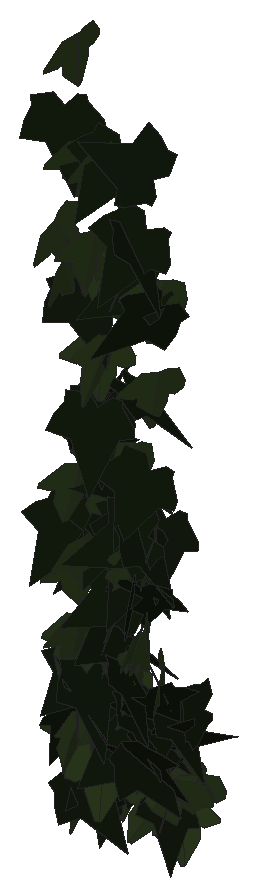
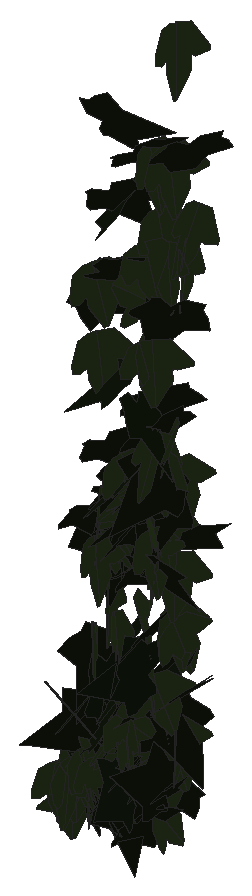
# SketchUp Ruby script. Lengths in inches.
U = 1.inch
M = Sketchup.active_model
def pt(a) = Geom::Point3d.new(a.map { |v| v * U })
def face(e, loops, mat)
  f = e.add_face(loops[0].map { |a| pt(a) })
  loops[1..].each { |l| e.add_face(l.map { |a| pt(a) }).erase! }
  f.material = f.back_material = mat if mat
  f
end
# faces: each face lists its corners as indices into pts; further lists are holes
def faces(e, pts, list, mat = nil) = list.each { |f| face(e, (f[0].is_a?(Array) ? f : [f]).map { |l| l.map { |i| pts[i] } }, mat) }
# xy, xz, yz: faces in a plane at the given z, y or x. An outline is a flat list of corners, or four numbers for a rectangle; further outlines are holes
def ring(l) = l.size == 4 ? [[l[0], l[1]], [l[2], l[1]], [l[2], l[3]], [l[0], l[3]]] : l.each_slice(2).to_a
def flat(e, list, mat, &to3) = list.each { |f| face(e, (f[0].is_a?(Array) ? f : [f]).map { |l| ring(l).map { |u, v| to3.(u, v) } }, mat) }
def xy(e, z, list, mat = nil) = flat(e, list, mat) { |x, y| [x, y, z] }
def xz(e, y, list, mat = nil) = flat(e, list, mat) { |x, z| [x, y, z] }
def yz(e, x, list, mat = nil) = flat(e, list, mat) { |y, z| [x, y, z] }
def lines(e, pts, list) = list.each { |a, b| e.add_line(pt(pts[a]), pt(pts[b])) }
# prism: a flat outline (further loops are holes) pulled along v
def prism(e, loops, v, mat = nil)
  f = face(e, loops, mat); d = Geom::Vector3d.new(v.map { |x| x * U })
  f.pushpull(f.normal.samedirection?(d) ? d.length : -d.length)
end
def box(e, o, s, mat = nil) = prism(e, [[o, [o[0] + s[0], o[1], o[2]], [o[0] + s[0], o[1] + s[1], o[2]], [o[0], o[1] + s[1], o[2]]]], [0, 0, s[2]], mat)
def at(x, y, z, deg = 0) = Geom::Transformation.translation(pt([x, y, z])) * Geom::Transformation.rotation(ORIGIN, Z_AXIS, deg.degrees)
def axes(o, x, y, z) = Geom::Transformation.new([*x, 0, *y, 0, *z, 0, *pt(o).to_a, 1])
def part(name) = M.definitions.add(name)
# library, detail: a bought-in or finely detailed component or shape, given as its bounding box
def library(name, o, s) = part(name).tap { |d| box(d.entities, o, s) }
def detail(e, o, s) = box(e.add_group.entities, o, s)
def put(e, d, t, mat = nil) = e.add_instance(d, t).tap { |i| i.material = mat if mat }
def group(e, t, mat = nil) = e.add_group.tap { |g| g.transformation = t; g.material = mat if mat }.entities
root = M.entities
M.materials.add("efeu1").color = [18, 25, 13]
M.materials.add("efeu2").color = [43, 57, 29]
c1 = part("ivyleaf_9")
p = [[1.54,2.16,1.25],[1.36,2.04,1.19],[-0.21,0.99,0.68],[-0.71,1.11,0.82],[-0.85,0.86,0.67],[-0.8,0.17,0.21],
  [-0.9,-0.01,0.1],[-0.67,-0.16,-0.02],[-0.08,-0.08,-0.05],[-0.03,-0.6,-0.4],[0.65,-0.88,-0.66],[0.83,-0.6,-0.49],
  [1.29,-0.42,-0.43],[1.8125,-0.07,-0.26],[1.21,0.44,0.15]]
faces(c1.entities,p,[[0,1,2,3,4,5,6,7,8,9,10,11,12,13,14]],"efeu1")
c2 = part("ivyleaf_10")
p = [[0,0.5,-0.03],[-0.0625,2.02,-0.43],[-0.19,2.01,-0.46],[-0.54,1.05,-0.29],[-0.52,0.625,-0.18],[-0.83,0.76,-0.28],
  [-1.16,0.64,-0.33],[-1.15,0.33,-0.24],[-0.77,-0.39,0.02],[-0.3,-0.51,0.16],[0.04,-0.48,0.23],[-0.02,2.01,-0.4375],
  [-0.06,2.01,-0.43],[0.04,-0.49,0.23],[0.67,-0.49,0.14],[1.38,0.36,-0.2],[1.375,0.51,-0.24],[0.81,0.65,-0.19],
  [0.62,0.59,-0.15],[0.6,1.09,-0.28],[0.5,1.23,-0.31]]
faces(c2.entities,p,[[0,1,2,3,4,5,6,7,8,9,10],[11,12,0,13,14,15,16,17,18,19,20]],"efeu2")
put(root,c1,axes([534.67,132.68,230.73],[-0.17047,-0.87063,-0.31313],[0.13235,0.29218,-0.88443],[0.91571,-0.2043,0.06954]))
put(root,c1,axes([535,132.6,216.09],[-0.49505,-0.70564,0.21497],[-0.01913,-0.24653,-0.85327],[0.73741,-0.48012,0.12218]))
put(root,c1,axes([534.84,133.875,207.48],[0.16353,0.01722,0.84757],[0.46903,0.71721,-0.10507],[-0.70617,0.48035,0.12649]))
put(root,c1,axes([535,133.2,210.3125],[-0.40753,-0.58007,0.50539],[-0.0202,-0.56365,-0.66322],[0.76908,-0.32218,0.25038]))
put(root,c2,axes([535.21,133.21,219.01],[-0.87167,0.19635,0.09667],[-0.12722,-0.13155,-0.8799],[-0.17809,-0.86709,0.15539]))
put(root,c2,axes([534.99,133.64,206.32],[0.17022,-0.68568,0.54442],[0.19711,-0.51036,-0.70442],[0.85305,0.25475,0.05413]))
put(root,c2,axes([535.3,133.59,210.88],[-0.51327,-0.62942,0.32203],[-0.08648,-0.33906,-0.80055],[0.70171,-0.50218,0.13689]))
put(root,c2,axes([535.08,133.01,220.08],[-0.46392,0.76914,-0.00582],[0.00287,-0.00506,-0.89822],[-0.76915,-0.46393,0.00015]))
put(root,c1,axes([535.41,132.59,209.51],[-0.00032,0.72675,-0.57082],[-0.0098,-0.5708,-0.7267],[-0.92407,0.00581,0.00791]))
put(root,c1,axes([535.11,134.04,206.78],[-0.27107,-0.63117,0.50294],[-0.07725,-0.50782,-0.67893],[0.80334,-0.26181,0.10441]))
put(root,c2,axes([535.51,132.76,208.73],[-0.64757,-0.66757,0.33135],[-0.19199,-0.27473,-0.92868],[0.72012,-0.67355,0.05038]))
put(root,c2,axes([535.35,133.72,216.23],[-0.13916,-0.88516,0.00004],[-0.00327,0.00047,-0.89602],[0.88515,-0.13916,-0.0033]))
put(root,c2,axes([535.4,132.28,208.78],[0.28299,-0.69072,-0.55775],[-0.1092,0.55387,-0.74132],[0.88105,0.2905,0.08727]))
put(root,c2,axes([535.33,132.43,212.42],[-0.20741,-0.77307,0.34276],[0.12229,-0.37663,-0.77545],[0.83676,-0.13658,0.19829]))
put(root,c1,axes([535.66,133.65,215.38],[-0.88423,-0.15992,-0.0197],[0.02107,-0.00578,-0.89853],[0.15975,-0.88443,0.00944]))
put(root,c2,axes([535.44,132.39,214.8125],[-0.42454,-0.77265,-0.09329],[0.03674,0.08625,-0.88156],[0.7774,-0.42603,-0.00928]))
put(root,c2,axes([535.34,131.5,227.28],[-0.08329,-0.81917,-0.55725],[0.1681,0.53942,-0.81809],[0.97638,-0.16275,0.09331]))
put(root,c1,axes([535.25,134.5,206.3],[-0.23027,-0.82502,0.03105],[-0.00851,-0.02986,-0.85655],[0.82556,-0.23043,-0.00017]))
put(root,c2,axes([535.54,132.21,218.11],[-0.34714,-0.81372,0.16705],[-0.036,-0.16614,-0.88411],[0.82991,-0.34758,0.03152]))
put(root,c1,axes([535.08,133.37,218.73],[0.80409,0.42348,0.0933],[0.09341,0.02278,-0.90849],[-0.42345,0.80917,-0.02325]))
put(root,c2,axes([535.59,132.48,229.77],[-0.32626,-0.89624,0.01194],[-0.00363,-0.01139,-0.95378],[0.89631,-0.32628,0.00049]))
put(root,c2,axes([535.53,133.26,215.76],[0.43509,-0.63287,-0.47452],[-0.04953,0.51871,-0.73722],[0.78946,0.38133,0.21527]))
put(root,c2,axes([535.55,131.54,225.99],[0.22422,-0.76891,-0.52224],[-0.01101,0.53498,-0.79241],[0.92943,0.19184,0.1166]))
put(root,c2,axes([535.58,132.16,212.76],[-0.13049,-0.88511,-0.01911],[0.001,0.01917,-0.89468],[0.88532,-0.13048,-0.0018]))
put(root,c2,axes([535.52,133.32,219.63],[-0.1619,-0.78602,-0.44335],[0.12954,0.42553,-0.80171],[0.89309,-0.20421,0.03592]))
put(root,c2,axes([535.53,133.54,217.13],[0.43022,-0.77724,0.17532],[0.07912,-0.15658,-0.88834],[0.79283,0.43738,-0.00648]))
put(root,c2,axes([535.91,132.37,226.08],[-0.85268,0.1476,0.327],[-0.33414,-0.01969,-0.8624],[-0.13064,-0.91302,0.07147]))
put(root,c1,axes([535.62,132.79,217.48],[0.66238,0.53861,-0.27147],[-0.244,-0.12946,-0.8522],[-0.5516,0.70405,0.05098]))
put(root,c2,axes([535.72,133.43,211.61],[0.51148,-0.64356,-0.29086],[-0.09639,0.29215,-0.81593],[0.69963,0.51074,0.10022]))
put(root,c1,axes([535.34,132.79,224.54],[-0.28565,-0.64315,-0.59252],[0.27511,0.52558,-0.70313],[0.83008,-0.39551,0.02914]))
put(root,c1,axes([535.8,134.68,207.38],[0.13468,0.46315,0.75382],[0.05072,0.7572,-0.4743],[-0.88328,0.1141,0.08771]))
put(root,c1,axes([536.08,133.48,220.95],[-0.52812,0.71989,-0.16553],[0.09619,-0.13473,-0.89283],[-0.73238,-0.5368,0.0021]))
put(root,c2,axes([535.81,131.86,233.93],[-0.1333,-0.94983,-0.2069],[0.02636,0.20523,-0.95914],[0.97175,-0.13586,-0.00236]))
put(root,c2,axes([535.95,134.45,209.92],[0.26425,0.58423,-0.62362],[-0.37411,-0.50779,-0.63424],[-0.76829,0.4482,0.09434]))
put(root,c2,axes([535.9375,134.1875,209.4],[0.56503,-0.5662,-0.32944],[-0.08799,0.36552,-0.77912],[0.64913,0.54239,0.18115]))
put(root,c1,axes([535.37,132.28,210.8],[0.50198,-0.68368,0.19339],[0.1189,-0.15261,-0.84816],[0.70049,0.51584,0.00538]))
put(root,c1,axes([535.66,133.22,220.25],[-0.08997,-0.9049,-0.15923],[-0.01163,0.1611,-0.90896],[0.91873,-0.08657,-0.0271]))
put(root,c1,axes([535.28,134.2,211.64],[0.81082,-0.25843,0.35026],[0.33924,-0.08882,-0.85084],[0.27273,0.87877,0.01701]))
put(root,c2,axes([535.58,132.89,209.71],[0.43676,-0.48327,0.57608],[0.50444,-0.30574,-0.63893],[0.55764,0.65509,0.12678]))
put(root,c2,axes([536.08,132.81,222.59],[-0.6913,-0.62824,0.08275],[0.06346,-0.19049,-0.91603],[0.63048,-0.66967,0.18293]))
put(root,c1,axes([536.3125,133.9375,206.54],[-0.0256,0.82399,-0.17062],[-0.01516,-0.17112,-0.82414],[-0.84133,-0.02199,0.02004]))
put(root,c1,axes([535.53,132.46,206.97],[-0.15224,-0.36617,-0.83759],[0.6488,0.55489,-0.36051],[0.64396,-0.64562,0.1652]))
put(root,c2,axes([536.17,133.9,208.81],[0.11068,-0.85815,0.05755],[0.01448,-0.05616,-0.86523],[0.85996,0.11139,0.00717]))
put(root,c2,axes([536.21,131.76,215.99],[-0.22414,-0.85782,-0.22933],[0.07823,0.21653,-0.88639],[0.88449,-0.23653,0.02028]))
put(root,c1,axes([536.18,133.39,216.4],[-0.53998,-0.72459,-0.00878],[0.00511,0.00714,-0.90366],[0.72462,-0.54001,-0.00017]))
put(root,c1,axes([535.81,133.93,209.71],[0.11803,-0.80548,-0.30843],[0.07201,0.31942,-0.80662],[0.8595,0.08385,0.10994]))
put(root,c1,axes([535.94,133.39,215.17],[-0.06778,-0.89999,0.09564],[-0.0165,-0.09467,-0.90249],[0.90491,-0.06914,-0.00929]))
put(root,c2,axes([536.3,132.8,226.12],[-0.56838,-0.69906,0.22096],[0.0126,-0.28886,-0.88146],[0.73304,-0.53706,0.18648]))
put(root,c2,axes([536.28,132.5,229.67],[-0.05331,-0.95011,-0.00492],[0.00252,0.00479,-0.9516],[0.95012,-0.05332,0.00225]))
put(root,c1,axes([536.16,133.54,212.15],[-0.28561,-0.5158,0.68147],[-0.12928,-0.68418,-0.57203],[0.84484,-0.27907,0.14284]))
put(root,c1,axes([535.86,134.82,207.79],[0.25489,-0.8035,0.04285],[0.00633,-0.04294,-0.84293],[0.80461,0.25488,-0.00694]))
put(root,c1,axes([536.73,133,210.33],[-0.08423,0.107,0.87489],[-0.38577,0.78575,-0.13324],[-0.79251,-0.39385,-0.02813]))
put(root,c2,axes([536.375,131.99,226.94],[-0.25014,-0.92495,0.04703],[-0.00874,-0.04636,-0.95817],[0.9261,-0.25027,0.00366]))
put(root,c1,axes([535.87,133.49,217.7],[-0.10174,-0.89325,0.00332],[0.31862,-0.03941,-0.83975],[0.8345,-0.09385,0.32103]))
put(root,c2,axes([536.32,133.11,213.16],[0.53984,-0.78008,-0.0211],[-0.01289,0.01674,-0.94865],[0.78026,0.53999,-0.00107]))
put(root,c2,axes([536.32,132.59,222.71],[-0.0005,-0.83337,0.44396],[0.1148,-0.44072,-0.82716],[0.93724,0.05353,0.10155]))
put(root,c2,axes([536.33,134.12,206.72],[0.65417,-0.54678,-0.05877],[-0.04133,0.04219,-0.85257],[0.54837,0.65544,0.00585]))
put(root,c1,axes([535.97,134.5,206.83],[-0.09155,-0.67542,0.52153],[0.24941,-0.5228,-0.63328],[0.81608,0.08401,0.25205]))
put(root,c1,axes([535.99,133.58,207.83],[0.21948,-0.58169,-0.59289],[0.00931,0.61492,-0.59986],[0.83054,0.14683,0.16341]))
put(root,c1,axes([535.99,132.14,210.99],[0.23034,-0.93145,-0.06282],[-0.01242,0.06165,-0.9595],[0.93349,0.23065,0.00274]))
put(root,c2,axes([536.57,133.58,218.59],[-0.36589,-0.79289,0.22799],[-0.00194,-0.24858,-0.8676],[0.82501,-0.35223,0.09907]))
put(root,c2,axes([536.26,132.54,207.9375],[0.94818,0.28216,0.07054],[0.06215,0.03843,-0.98908],[-0.28413,0.95002,0.01905]))
put(root,c1,axes([536.34,132.22,220.66],[-0.38329,-0.82169,-0.24492],[0.10314,0.22214,-0.90669],[0.85119,-0.39692,-0.00043]))
put(root,c1,axes([536.09,133.26,218.05],[0.31573,-0.84954,-0.04702],[0.04089,0.06525,-0.90426],[0.84985,0.31248,0.06097]))
put(root,c2,axes([536.22,132.73,217.7],[-0.04594,-0.42333,-0.93647],[0.52581,0.79574,-0.38551],[0.88301,-0.49587,0.18084]))
put(root,c1,axes([536.27,133.47,207.75],[0.66458,-0.46572,-0.27422],[-0.14814,0.26102,-0.8023],[0.51976,0.66987,0.12196]))
put(root,c2,axes([536.72,132.85,224.48],[0.34283,-0.52953,0.67862],[-0.2841,0.61992,0.62725],[-0.81253,-0.44017,0.06701]))
put(root,c1,axes([536.28,133.4,218.6],[0.6609,-0.51762,-0.33874],[-0.12465,0.3741,-0.81485],[0.60592,0.64155,0.20184]))
put(root,c1,axes([536.35,134.25,207.16],[0.24742,-0.81913,-0.07357],[0.01555,0.08147,-0.85483],[0.82228,0.24493,0.0383]))
put(root,c1,axes([536.36,132.74,216.54],[0.52809,-0.54388,-0.48464],[-0.14215,0.51015,-0.72739],[0.71447,0.50349,0.21349]))
put(root,c2,axes([536.86,134.44,207.75],[-0.59421,-0.60841,0.14157],[0.03327,-0.22595,-0.83135],[0.62378,-0.56752,0.17921]))
put(root,c1,axes([536.79,132.73,229.8],[-0.53907,-0.73004,0.21783],[-0.00018,-0.26672,-0.89435],[0.76185,-0.51662,0.15392]))
put(root,c2,axes([536.67,133.33,209.13],[0.13613,-0.56883,-0.73164],[0.32508,0.72182,-0.50071],[0.86787,-0.18114,0.30232]))
put(root,c1,axes([537.13,132.99,207.76],[0.31857,0.61112,-0.55909],[-0.34288,-0.44798,-0.68505],[-0.75398,0.46193,0.0753]))
put(root,c1,axes([537.2,132.6,214.08],[-0.6451,-0.36134,0.48606],[-0.16709,-0.57639,-0.65026],[0.58215,-0.56585,0.35198]))
put(root,c2,axes([537.14,133.26,212.38],[0.2608,-0.79449,-0.28458],[-0.06009,0.27962,-0.83571],[0.84178,0.26611,0.02851]))
put(root,c2,axes([536.82,133.5625,210.88],[-0.01411,-0.38893,0.80756],[0.49409,-0.67724,-0.31753],[0.74785,0.4401,0.22502]))
put(root,c1,axes([537.89,134.15,206.48],[-0.36706,0.03281,-0.83347],[-0.83224,-0.07533,0.36356],[-0.0558,0.90759,0.0603]))
put(root,c1,axes([537.21,132.62,208.63],[-0.4531,-0.55381,0.54649],[-0.05666,-0.60725,-0.66235],[0.77598,-0.36771,0.27074]))
put(root,c1,axes([537.64,133.36,225.33],[-0.71728,-0.35723,0.44081],[-0.34469,-0.29003,-0.79592],[0.45069,-0.79037,0.09283]))
put(root,c2,axes([537.38,134.03,215.4375],[-0.02771,-0.87059,-0.14113],[-0.00278,0.14129,-0.871],[0.88195,-0.02691,-0.00718]))
put(root,c1,axes([536.79,134.43,210.46],[0.16594,-0.40279,0.79125],[0.32629,-0.72095,-0.43544],[0.82574,0.36583,0.01305]))
put(root,c1,axes([537.04,133.57,208.58],[0.6839,-0.47552,-0.21419],[-0.11054,0.21303,-0.8259],[0.50968,0.68426,0.10828]))
put(root,c2,axes([537.58,134.48,207.72],[-0.04912,-0.8447,0.12551],[-0.02883,-0.12401,-0.84585],[0.85348,-0.0528,-0.02135]))
put(root,c2,axes([537.88,134.36,207.98],[-0.78457,0.16122,0.32304],[-0.33763,-0.05396,-0.79309],[-0.12786,-0.84676,0.11204]))
put(root,c1,axes([537.2,132.53,216.79],[0.05576,-0.67564,-0.60536],[0.11113,0.60703,-0.66726],[0.90034,-0.03308,0.11986]))
put(root,c2,axes([537.57,132.5625,215.29],[0.04669,-0.79996,0.47142],[0.14744,-0.45964,-0.79457],[0.91676,0.11466,0.10378]))
put(root,c1,axes([538.22,132.26,216.76],[-0.80991,-0.14502,0.48085],[-0.4737,-0.08261,-0.82279],[0.16689,-0.93827,-0.00187]))
put(root,c2,axes([537.65,133.11,208.27],[0.33509,-0.71241,-0.32832],[0.00276,0.35809,-0.77419],[0.78442,0.30307,0.14298]))
put(root,c1,axes([537.24,133.18,215.95],[0.27043,-0.83253,-0.26467],[0.00998,0.27999,-0.87051],[0.87353,0.25454,0.09189]))
put(root,c1,axes([537.19,133,209.9],[0.43115,-0.74571,0.10087],[0.05913,-0.08233,-0.86132],[0.75018,0.43507,0.00991]))
put(root,c1,axes([538.01,133.625,207.5],[-0.37262,0.74438,-0.22777],[0.06991,-0.2195,-0.83171],[-0.7753,-0.37755,0.03448]))
put(root,c1,axes([537.11,132.875,221.51],[0.75696,-0.53989,-0.11564],[0.06185,0.27791,-0.89262],[0.54866,0.71353,0.26017]))
put(root,c1,axes([537.69,132.74,215.62],[-0.39628,-0.79037,0.17718],[-0.05253,-0.17176,-0.88366],[0.80829,-0.39866,0.02944]))
put(root,c1,axes([537.39,133.62,208.86],[0.70246,-0.35338,-0.35224],[-0.19499,0.36548,-0.75552],[0.45928,0.69566,0.218]))
put(root,c2,axes([537.86,132.47,215.86],[-0.05145,-0.72878,0.5131],[0.04015,-0.51532,-0.72791],[0.89038,-0.01888,0.06247]))
put(root,c2,axes([538.13,133.09,206.83],[-0.54347,-0.41349,0.48166],[-0.25159,-0.44184,-0.66318],[0.58281,-0.57631,0.16286]))
put(root,c1,axes([538.15,133.03,224.65],[-0.13363,0.15373,-0.90287],[0.0112,-0.91209,-0.15696],[-0.9158,-0.03359,0.12983]))
put(root,c1,axes([538.625,132,229.95],[-0.38468,0.23685,0.83177],[-0.80053,0.24695,-0.44056],[-0.32725,-0.88252,0.09995]))
put(root,c1,axes([537.36,132.42,211.33],[0.35829,-0.74519,0.28542],[0.13704,-0.25077,-0.82673],[0.78613,0.38335,0.01403]))
put(root,c2,axes([538,133.34,225.05],[-0.4706,-0.75334,0.21424],[-0.00689,-0.24595,-0.87997],[0.78319,-0.45483,0.12099]))
put(root,c2,axes([538.05,133.71,206.8125],[0.33839,-0.6322,-0.47254],[-0.16982,0.44378,-0.71533],[0.7708,0.37532,0.04986]))
put(root,c1,axes([537.93,132.77,218.71],[-0.53488,-0.73896,0.00026],[-0.02288,0.01623,-0.91179],[0.73861,-0.53463,-0.02805]))
put(root,c2,axes([538.12,134.67,207.1],[-0.80906,0.15739,0.19616],[-0.18979,0.05153,-0.82411],[-0.16502,-0.83091,-0.01395]))
put(root,c1,axes([538.15,131.53,214.14],[0.08056,-0.05162,0.99681],[0.06461,0.99823,0.04647],[-0.99605,0.06058,0.08364]))
put(root,c1,axes([538.1,132.35,227.66],[-0.71967,-0.61543,0.00391],[-0.00296,-0.00255,-0.94693],[0.61543,-0.71967,0.00001]))
put(root,c2,axes([538.03,132.43,213.04],[0.28868,-0.77771,-0.35117],[0.01671,0.3758,-0.81852],[0.85315,0.25579,0.13485]))
put(root,c2,axes([538.16,132.76,216.27],[0.30846,-0.76378,-0.61823],[-0.08286,0.62545,-0.81405],[0.97913,0.29355,0.12587]))
put(root,c1,axes([537.75,132.03,208.92],[0.96867,0.26593,0.01271],[0.01222,0.0035,-1.00451],[-0.26596,0.96875,0.00014]))
put(root,c2,axes([538.27,132.83,222.14],[-0.41021,-0.82132,0.04236],[-0.01506,-0.03983,-0.91806],[0.82228,-0.41047,0.00432]))
put(root,c2,axes([538.24,133.05,211.5],[0.4397,-0.68279,-0.43084],[-0.08914,0.44654,-0.79864],[0.80242,0.42375,0.14737]))
put(root,c1,axes([537.89,132.31,208.93],[0.27851,-0.62861,-0.64979],[-0.19746,0.62122,-0.6856],[0.88226,0.33748,0.05168]))
put(root,c1,axes([538,133.55,216.64],[-0.23977,-0.85714,-0.10271],[0.02136,0.10067,-0.89002],[0.86301,-0.24063,-0.0065]))
put(root,c2,axes([538.36,134,206.94],[-0.73933,-0.37225,0.10008],[-0.08953,-0.04472,-0.82775],[0.37492,-0.74473,-0.00032]))
put(root,c1,axes([538.37,131.91,215.07],[0.52393,0.57705,-0.44003],[-0.39622,-0.22722,-0.76973],[-0.60796,0.64537,0.12244]))
put(root,c2,axes([538.16,134.63,207.17],[-0.12095,-0.68836,0.4772],[0.17001,-0.49229,-0.66703],[0.82015,0.00053,0.20865]))
put(root,c1,axes([538.17,132.47,210.84],[0.50005,0.74234,0.01204],[0.00374,0.012,-0.89504],[-0.74242,0.50005,0.0036]))
put(root,c1,axes([537.73,132.26,227.32],[0.43209,-0.81822,0.1464],[0.08685,-0.11966,-0.92507],[0.82666,0.44024,0.02066]))
put(root,c1,axes([537.82,133.62,208.65],[0.5634,0.25057,0.59872],[0.47969,0.37331,-0.60762],[-0.43721,0.73248,0.10486]))
put(root,c1,axes([538.08,133.75,206.54],[0.00907,-0.83001,0.03306],[0.00053,-0.03305,-0.83006],[0.83067,0.00909,0.00017]))
put(root,c1,axes([538,132.24,216.86],[0.42015,-0.74213,-0.27037],[-0.08424,0.26239,-0.85114],[0.78534,0.42518,0.05334]))
put(root,c2,axes([538.23,134.12,206.04],[0.55168,0.64521,0.02485],[0.0211,0.01465,-0.84888],[-0.64534,0.55205,-0.00652]))
put(root,c1,axes([538.84,134.35,209.8],[-0.79564,0.28436,-0.02191],[0.0133,-0.02785,-0.84465],[-0.28489,-0.79546,0.02175]))
put(root,c1,axes([537.97,133.99,209.61],[0.42044,-0.76253,-0.03422],[0.04224,0.06225,-0.86818],[0.76212,0.41721,0.06699]))
put(root,c2,axes([538.57,134.46,206.95],[-0.56057,-0.6392,0.08068],[0.02735,-0.13046,-0.84354],[0.6437,-0.55111,0.1061]))
